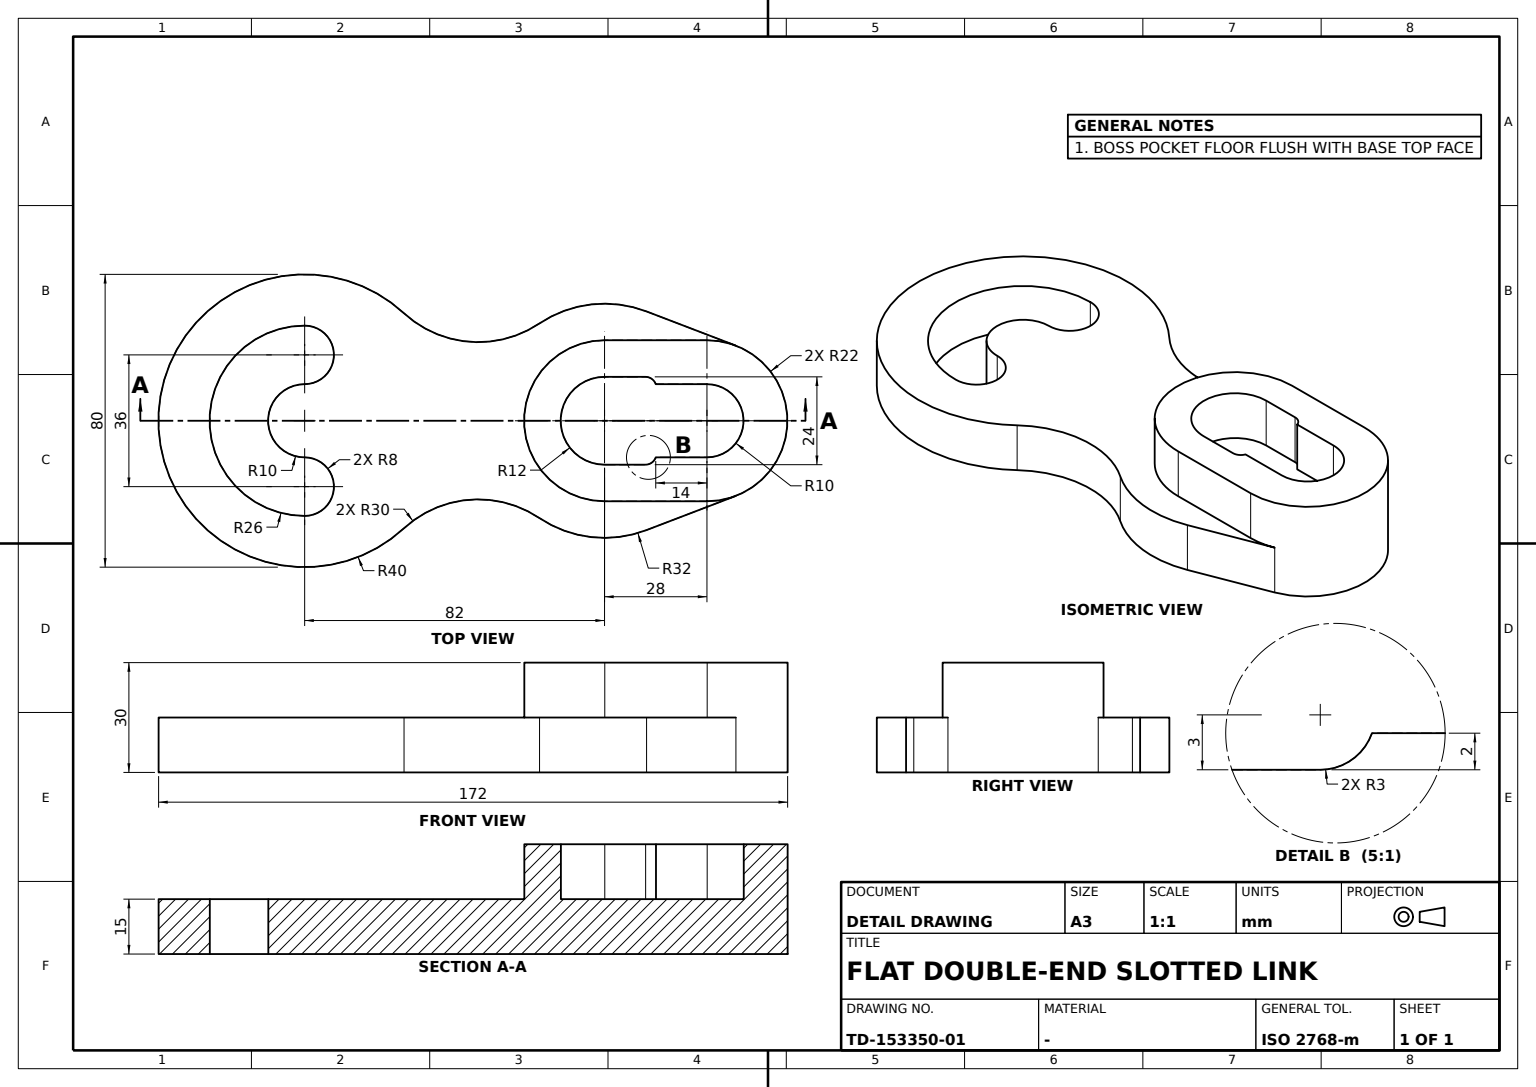
ISO-10303-21;
HEADER;
FILE_DESCRIPTION((''),'2;1');
FILE_NAME('','',(''),(''),'','','');
FILE_SCHEMA(('AUTOMOTIVE_DESIGN'));
ENDSEC;
DATA;
#1=APPLICATION_CONTEXT('');
#2=PRODUCT_CONTEXT('',#1,'mechanical');
#3=PRODUCT('','','',(#2));
#4=PRODUCT_DEFINITION_FORMATION('','',#3);
#5=PRODUCT_DEFINITION_CONTEXT('',#1,'design');
#6=PRODUCT_DEFINITION('','',#4,#5);
#7=PRODUCT_DEFINITION_SHAPE('','',#6);
#8=(LENGTH_UNIT()NAMED_UNIT(*)SI_UNIT(.MILLI.,.METRE.));
#9=(NAMED_UNIT(*)PLANE_ANGLE_UNIT()SI_UNIT($,.RADIAN.));
#10=(NAMED_UNIT(*)SI_UNIT($,.STERADIAN.)SOLID_ANGLE_UNIT());
#11=UNCERTAINTY_MEASURE_WITH_UNIT(LENGTH_MEASURE(0.005),#8,'distance_accuracy_value','');
#12=(GEOMETRIC_REPRESENTATION_CONTEXT(3)GLOBAL_UNCERTAINTY_ASSIGNED_CONTEXT((#11))GLOBAL_UNIT_ASSIGNED_CONTEXT((#8,#9,#10))REPRESENTATION_CONTEXT('',''));
#13=CARTESIAN_POINT('',(-10.,110.,15.));
#14=VERTEX_POINT('',#13);
#15=CARTESIAN_POINT('',(-10.,96.,15.));
#16=VERTEX_POINT('',#15);
#17=CARTESIAN_POINT('',(-10.,0.,15.));
#18=DIRECTION('',(0.,-1.,0.));
#19=VECTOR('',#18,1000.);
#20=LINE('',#17,#19);
#21=EDGE_CURVE('',#14,#16,#20,.T.);
#22=ORIENTED_EDGE('',*,*,#21,.T.);
#23=CARTESIAN_POINT('',(-10.,96.,0.));
#24=VERTEX_POINT('',#23);
#25=DIRECTION('',(0.,0.,1.));
#26=VECTOR('',#25,1000.);
#27=LINE('',#23,#26);
#28=EDGE_CURVE('',#24,#16,#27,.T.);
#29=ORIENTED_EDGE('',*,*,#28,.F.);
#30=CARTESIAN_POINT('',(-10.,110.,0.));
#31=VERTEX_POINT('',#30);
#32=CARTESIAN_POINT('',(-10.,0.,0.));
#33=LINE('',#32,#19);
#34=EDGE_CURVE('',#31,#24,#33,.T.);
#35=ORIENTED_EDGE('',*,*,#34,.F.);
#36=CARTESIAN_POINT('',(-10.,110.,7.5));
#37=LINE('',#36,#26);
#38=EDGE_CURVE('',#31,#14,#37,.T.);
#39=ORIENTED_EDGE('',*,*,#38,.T.);
#40=EDGE_LOOP('',(#22,#29,#35,#39));
#41=FACE_BOUND('',#40,.T.);
#42=DIRECTION('',(-1.,0.,0.));
#43=AXIS2_PLACEMENT_3D('',#30,#42,#18);
#44=PLANE('',#43);
#45=ADVANCED_FACE('',(#41),#44,.F.);
#46=CARTESIAN_POINT('',(12.,93.171573,0.));
#47=VERTEX_POINT('',#46);
#48=CARTESIAN_POINT('',(10.,96.,0.));
#49=VERTEX_POINT('',#48);
#50=CARTESIAN_POINT('',(9.,93.171573,0.));
#51=DIRECTION('',(1.,0.,0.));
#52=AXIS2_PLACEMENT_3D('',#50,#25,#51);
#53=CIRCLE('',#52,3.);
#54=EDGE_CURVE('',#47,#49,#53,.T.);
#55=ORIENTED_EDGE('',*,*,#54,.F.);
#56=CARTESIAN_POINT('',(12.,93.171573,15.));
#57=VERTEX_POINT('',#56);
#58=CARTESIAN_POINT('',(12.,93.171573,7.5));
#59=LINE('',#58,#26);
#60=EDGE_CURVE('',#47,#57,#59,.T.);
#61=ORIENTED_EDGE('',*,*,#60,.T.);
#62=CARTESIAN_POINT('',(10.,96.,15.));
#63=VERTEX_POINT('',#62);
#64=CARTESIAN_POINT('',(9.,93.171573,15.));
#65=AXIS2_PLACEMENT_3D('',#64,#25,#51);
#66=CIRCLE('',#65,3.);
#67=EDGE_CURVE('',#57,#63,#66,.T.);
#68=ORIENTED_EDGE('',*,*,#67,.T.);
#69=LINE('',#48,#26);
#70=EDGE_CURVE('',#49,#63,#69,.T.);
#71=ORIENTED_EDGE('',*,*,#70,.F.);
#72=EDGE_LOOP('',(#55,#61,#68,#71));
#73=FACE_BOUND('',#72,.T.);
#74=CARTESIAN_POINT('',(9.,93.171573,7.5));
#75=AXIS2_PLACEMENT_3D('',#74,#25,#51);
#76=CYLINDRICAL_SURFACE('',#75,3.);
#77=ADVANCED_FACE('',(#73),#76,.F.);
#78=ORIENTED_EDGE('',*,*,#34,.T.);
#79=CARTESIAN_POINT('',(-12.,93.171573,0.));
#80=VERTEX_POINT('',#79);
#81=CARTESIAN_POINT('',(-9.,93.171573,0.));
#82=AXIS2_PLACEMENT_3D('',#81,#25,#51);
#83=CIRCLE('',#82,3.);
#84=EDGE_CURVE('',#24,#80,#83,.T.);
#85=ORIENTED_EDGE('',*,*,#84,.T.);
#86=CARTESIAN_POINT('',(-12.,82.,0.));
#87=VERTEX_POINT('',#86);
#88=CARTESIAN_POINT('',(-12.,0.,0.));
#89=DIRECTION('',(0.,1.,0.));
#90=VECTOR('',#89,1000.);
#91=LINE('',#88,#90);
#92=EDGE_CURVE('',#87,#80,#91,.T.);
#93=ORIENTED_EDGE('',*,*,#92,.F.);
#94=CARTESIAN_POINT('',(12.,82.,0.));
#95=VERTEX_POINT('',#94);
#96=CARTESIAN_POINT('',(0.,82.,0.));
#97=AXIS2_PLACEMENT_3D('',#96,#25,#51);
#98=CIRCLE('',#97,12.);
#99=EDGE_CURVE('',#87,#95,#98,.T.);
#100=ORIENTED_EDGE('',*,*,#99,.T.);
#101=CARTESIAN_POINT('',(12.,0.,0.));
#102=LINE('',#101,#90);
#103=EDGE_CURVE('',#95,#47,#102,.T.);
#104=ORIENTED_EDGE('',*,*,#103,.T.);
#105=ORIENTED_EDGE('',*,*,#54,.T.);
#106=CARTESIAN_POINT('',(10.,110.,0.));
#107=VERTEX_POINT('',#106);
#108=CARTESIAN_POINT('',(10.,0.,0.));
#109=LINE('',#108,#19);
#110=EDGE_CURVE('',#107,#49,#109,.T.);
#111=ORIENTED_EDGE('',*,*,#110,.F.);
#112=CARTESIAN_POINT('',(0.,110.,0.));
#113=AXIS2_PLACEMENT_3D('',#112,#25,#51);
#114=CIRCLE('',#113,10.);
#115=EDGE_CURVE('',#107,#31,#114,.T.);
#116=ORIENTED_EDGE('',*,*,#115,.T.);
#117=EDGE_LOOP('',(#78,#85,#93,#100,#104,#105,#111,#116));
#118=FACE_BOUND('',#117,.T.);
#119=CARTESIAN_POINT('',(0.,0.,0.));
#120=AXIS2_PLACEMENT_3D('',#119,#25,#51);
#121=PLANE('',#120);
#122=ADVANCED_FACE('',(#118),#121,.T.);
#123=CARTESIAN_POINT('',(-29.413527,27.108014,0.));
#124=VERTEX_POINT('',#123);
#125=CARTESIAN_POINT('',(-26.567057,64.162077,0.));
#126=VERTEX_POINT('',#125);
#127=CARTESIAN_POINT('',(-51.473673,47.439024,0.));
#128=AXIS2_PLACEMENT_3D('',#127,#25,#51);
#129=CIRCLE('',#128,30.);
#130=EDGE_CURVE('',#124,#126,#129,.T.);
#131=ORIENTED_EDGE('',*,*,#130,.T.);
#132=CARTESIAN_POINT('',(-26.567057,64.162077,-15.));
#133=VERTEX_POINT('',#132);
#134=CARTESIAN_POINT('',(-26.567057,64.162077,-7.5));
#135=LINE('',#134,#26);
#136=EDGE_CURVE('',#126,#133,#135,.F.);
#137=ORIENTED_EDGE('',*,*,#136,.T.);
#138=CARTESIAN_POINT('',(-29.413527,27.108014,-15.));
#139=VERTEX_POINT('',#138);
#140=CARTESIAN_POINT('',(-51.473673,47.439024,-15.));
#141=AXIS2_PLACEMENT_3D('',#140,#25,#51);
#142=CIRCLE('',#141,30.);
#143=EDGE_CURVE('',#139,#133,#142,.T.);
#144=ORIENTED_EDGE('',*,*,#143,.F.);
#145=CARTESIAN_POINT('',(-29.413527,27.108014,-7.5));
#146=LINE('',#145,#26);
#147=EDGE_CURVE('',#124,#139,#146,.F.);
#148=ORIENTED_EDGE('',*,*,#147,.F.);
#149=EDGE_LOOP('',(#131,#137,#144,#148));
#150=FACE_BOUND('',#149,.T.);
#151=CARTESIAN_POINT('',(-51.473673,47.439024,-7.5));
#152=AXIS2_PLACEMENT_3D('',#151,#25,#51);
#153=CYLINDRICAL_SURFACE('',#152,30.);
#154=ADVANCED_FACE('',(#150),#153,.F.);
#155=CARTESIAN_POINT('',(29.889593,93.428571,0.));
#156=VERTEX_POINT('',#155);
#157=CARTESIAN_POINT('',(20.549095,117.857143,0.));
#158=VERTEX_POINT('',#157);
#159=DIRECTION('',(-0.357142857,0.934049774,0.));
#160=VECTOR('',#159,1000.);
#161=LINE('',#155,#160);
#162=EDGE_CURVE('',#156,#158,#161,.T.);
#163=ORIENTED_EDGE('',*,*,#162,.F.);
#164=CARTESIAN_POINT('',(29.889593,93.428571,-15.));
#165=VERTEX_POINT('',#164);
#166=CARTESIAN_POINT('',(29.889593,93.428571,-7.5));
#167=LINE('',#166,#26);
#168=EDGE_CURVE('',#156,#165,#167,.F.);
#169=ORIENTED_EDGE('',*,*,#168,.T.);
#170=CARTESIAN_POINT('',(20.549095,117.857143,-15.));
#171=VERTEX_POINT('',#170);
#172=LINE('',#164,#160);
#173=EDGE_CURVE('',#165,#171,#172,.T.);
#174=ORIENTED_EDGE('',*,*,#173,.T.);
#175=CARTESIAN_POINT('',(20.549095,117.857143,-7.5));
#176=LINE('',#175,#26);
#177=EDGE_CURVE('',#158,#171,#176,.F.);
#178=ORIENTED_EDGE('',*,*,#177,.F.);
#179=EDGE_LOOP('',(#163,#169,#174,#178));
#180=FACE_BOUND('',#179,.T.);
#181=DIRECTION('',(-0.934049774,-0.357142857,0.));
#182=AXIS2_PLACEMENT_3D('',#155,#181,#159);
#183=PLANE('',#182);
#184=ADVANCED_FACE('',(#180),#183,.F.);
#185=CARTESIAN_POINT('',(-22.,82.,0.));
#186=VERTEX_POINT('',#185);
#187=CARTESIAN_POINT('',(-22.,82.,15.));
#188=VERTEX_POINT('',#187);
#189=CARTESIAN_POINT('',(-22.,82.,7.5));
#190=LINE('',#189,#26);
#191=EDGE_CURVE('',#186,#188,#190,.T.);
#192=ORIENTED_EDGE('',*,*,#191,.T.);
#193=CARTESIAN_POINT('',(-22.,110.,15.));
#194=VERTEX_POINT('',#193);
#195=CARTESIAN_POINT('',(-22.,0.,15.));
#196=LINE('',#195,#90);
#197=EDGE_CURVE('',#188,#194,#196,.T.);
#198=ORIENTED_EDGE('',*,*,#197,.T.);
#199=CARTESIAN_POINT('',(-22.,110.,0.));
#200=VERTEX_POINT('',#199);
#201=CARTESIAN_POINT('',(-22.,110.,-7.5));
#202=LINE('',#201,#26);
#203=EDGE_CURVE('',#200,#194,#202,.T.);
#204=ORIENTED_EDGE('',*,*,#203,.F.);
#205=CARTESIAN_POINT('',(-22.,0.,0.));
#206=LINE('',#205,#90);
#207=EDGE_CURVE('',#186,#200,#206,.T.);
#208=ORIENTED_EDGE('',*,*,#207,.F.);
#209=EDGE_LOOP('',(#192,#198,#204,#208));
#210=FACE_BOUND('',#209,.T.);
#211=AXIS2_PLACEMENT_3D('',#185,#51,#89);
#212=PLANE('',#211);
#213=ADVANCED_FACE('',(#210),#212,.F.);
#214=ORIENTED_EDGE('',*,*,#168,.F.);
#215=CARTESIAN_POINT('',(26.567057,64.162077,0.));
#216=VERTEX_POINT('',#215);
#217=CIRCLE('',#97,32.);
#218=EDGE_CURVE('',#216,#156,#217,.T.);
#219=ORIENTED_EDGE('',*,*,#218,.F.);
#220=CARTESIAN_POINT('',(26.567057,64.162077,-15.));
#221=VERTEX_POINT('',#220);
#222=CARTESIAN_POINT('',(26.567057,64.162077,-7.5));
#223=LINE('',#222,#26);
#224=EDGE_CURVE('',#216,#221,#223,.F.);
#225=ORIENTED_EDGE('',*,*,#224,.T.);
#226=CARTESIAN_POINT('',(0.,82.,-15.));
#227=AXIS2_PLACEMENT_3D('',#226,#25,#51);
#228=CIRCLE('',#227,32.);
#229=EDGE_CURVE('',#221,#165,#228,.T.);
#230=ORIENTED_EDGE('',*,*,#229,.T.);
#231=EDGE_LOOP('',(#214,#219,#225,#230));
#232=FACE_BOUND('',#231,.T.);
#233=CARTESIAN_POINT('',(0.,82.,-7.5));
#234=AXIS2_PLACEMENT_3D('',#233,#25,#51);
#235=CYLINDRICAL_SURFACE('',#234,32.);
#236=ADVANCED_FACE('',(#232),#235,.T.);
#237=CARTESIAN_POINT('',(26.,0.,0.));
#238=VERTEX_POINT('',#237);
#239=CARTESIAN_POINT('',(26.,0.,-15.));
#240=VERTEX_POINT('',#239);
#241=CARTESIAN_POINT('',(26.,0.,-7.5));
#242=LINE('',#241,#26);
#243=EDGE_CURVE('',#238,#240,#242,.F.);
#244=ORIENTED_EDGE('',*,*,#243,.F.);
#245=VERTEX_POINT('',#108);
#246=CARTESIAN_POINT('',(18.,0.,0.));
#247=AXIS2_PLACEMENT_3D('',#246,#25,#51);
#248=CIRCLE('',#247,8.);
#249=EDGE_CURVE('',#238,#245,#248,.T.);
#250=ORIENTED_EDGE('',*,*,#249,.T.);
#251=CARTESIAN_POINT('',(10.,0.,-15.));
#252=VERTEX_POINT('',#251);
#253=CARTESIAN_POINT('',(10.,0.,-7.5));
#254=LINE('',#253,#26);
#255=EDGE_CURVE('',#245,#252,#254,.F.);
#256=ORIENTED_EDGE('',*,*,#255,.T.);
#257=CARTESIAN_POINT('',(18.,0.,-15.));
#258=AXIS2_PLACEMENT_3D('',#257,#25,#51);
#259=CIRCLE('',#258,8.);
#260=EDGE_CURVE('',#240,#252,#259,.T.);
#261=ORIENTED_EDGE('',*,*,#260,.F.);
#262=EDGE_LOOP('',(#244,#250,#256,#261));
#263=FACE_BOUND('',#262,.T.);
#264=CARTESIAN_POINT('',(18.,0.,-7.5));
#265=AXIS2_PLACEMENT_3D('',#264,#25,#51);
#266=CYLINDRICAL_SURFACE('',#265,8.);
#267=ADVANCED_FACE('',(#263),#266,.F.);
#268=ORIENTED_EDGE('',*,*,#191,.F.);
#269=CARTESIAN_POINT('',(22.,82.,0.));
#270=VERTEX_POINT('',#269);
#271=CIRCLE('',#97,22.);
#272=EDGE_CURVE('',#186,#270,#271,.T.);
#273=ORIENTED_EDGE('',*,*,#272,.T.);
#274=CARTESIAN_POINT('',(22.,82.,15.));
#275=VERTEX_POINT('',#274);
#276=CARTESIAN_POINT('',(22.,82.,7.5));
#277=LINE('',#276,#26);
#278=EDGE_CURVE('',#270,#275,#277,.T.);
#279=ORIENTED_EDGE('',*,*,#278,.T.);
#280=CARTESIAN_POINT('',(0.,82.,15.));
#281=AXIS2_PLACEMENT_3D('',#280,#25,#51);
#282=CIRCLE('',#281,22.);
#283=EDGE_CURVE('',#188,#275,#282,.T.);
#284=ORIENTED_EDGE('',*,*,#283,.F.);
#285=EDGE_LOOP('',(#268,#273,#279,#284));
#286=FACE_BOUND('',#285,.T.);
#287=CARTESIAN_POINT('',(0.,82.,7.5));
#288=AXIS2_PLACEMENT_3D('',#287,#25,#51);
#289=CYLINDRICAL_SURFACE('',#288,22.);
#290=ADVANCED_FACE('',(#286),#289,.T.);
#291=CARTESIAN_POINT('',(29.413527,27.108014,0.));
#292=VERTEX_POINT('',#291);
#293=CARTESIAN_POINT('',(29.413527,27.108014,-15.));
#294=VERTEX_POINT('',#293);
#295=CARTESIAN_POINT('',(29.413527,27.108014,-7.5));
#296=LINE('',#295,#26);
#297=EDGE_CURVE('',#292,#294,#296,.F.);
#298=ORIENTED_EDGE('',*,*,#297,.T.);
#299=CARTESIAN_POINT('',(51.473673,47.439024,-15.));
#300=AXIS2_PLACEMENT_3D('',#299,#25,#51);
#301=CIRCLE('',#300,30.);
#302=EDGE_CURVE('',#221,#294,#301,.T.);
#303=ORIENTED_EDGE('',*,*,#302,.F.);
#304=ORIENTED_EDGE('',*,*,#224,.F.);
#305=CARTESIAN_POINT('',(51.473673,47.439024,0.));
#306=AXIS2_PLACEMENT_3D('',#305,#25,#51);
#307=CIRCLE('',#306,30.);
#308=EDGE_CURVE('',#216,#292,#307,.T.);
#309=ORIENTED_EDGE('',*,*,#308,.T.);
#310=EDGE_LOOP('',(#298,#303,#304,#309));
#311=FACE_BOUND('',#310,.T.);
#312=CARTESIAN_POINT('',(51.473673,47.439024,-7.5));
#313=AXIS2_PLACEMENT_3D('',#312,#25,#51);
#314=CYLINDRICAL_SURFACE('',#313,30.);
#315=ADVANCED_FACE('',(#311),#314,.F.);
#316=ORIENTED_EDGE('',*,*,#110,.T.);
#317=ORIENTED_EDGE('',*,*,#70,.T.);
#318=CARTESIAN_POINT('',(10.,110.,15.));
#319=VERTEX_POINT('',#318);
#320=CARTESIAN_POINT('',(10.,0.,15.));
#321=LINE('',#320,#19);
#322=EDGE_CURVE('',#319,#63,#321,.T.);
#323=ORIENTED_EDGE('',*,*,#322,.F.);
#324=CARTESIAN_POINT('',(10.,110.,7.5));
#325=LINE('',#324,#26);
#326=EDGE_CURVE('',#107,#319,#325,.T.);
#327=ORIENTED_EDGE('',*,*,#326,.F.);
#328=EDGE_LOOP('',(#316,#317,#323,#327));
#329=FACE_BOUND('',#328,.T.);
#330=AXIS2_PLACEMENT_3D('',#106,#42,#18);
#331=PLANE('',#330);
#332=ADVANCED_FACE('',(#329),#331,.T.);
#333=ORIENTED_EDGE('',*,*,#103,.F.);
#334=CARTESIAN_POINT('',(12.,82.,15.));
#335=VERTEX_POINT('',#334);
#336=CARTESIAN_POINT('',(12.,82.,7.5));
#337=LINE('',#336,#26);
#338=EDGE_CURVE('',#95,#335,#337,.T.);
#339=ORIENTED_EDGE('',*,*,#338,.T.);
#340=CARTESIAN_POINT('',(12.,0.,15.));
#341=LINE('',#340,#90);
#342=EDGE_CURVE('',#335,#57,#341,.T.);
#343=ORIENTED_EDGE('',*,*,#342,.T.);
#344=ORIENTED_EDGE('',*,*,#60,.F.);
#345=EDGE_LOOP('',(#333,#339,#343,#344));
#346=FACE_BOUND('',#345,.T.);
#347=AXIS2_PLACEMENT_3D('',#94,#51,#89);
#348=PLANE('',#347);
#349=ADVANCED_FACE('',(#346),#348,.F.);
#350=VERTEX_POINT('',#32);
#351=CARTESIAN_POINT('',(-10.,0.,-15.));
#352=VERTEX_POINT('',#351);
#353=CARTESIAN_POINT('',(-10.,0.,-7.5));
#354=LINE('',#353,#26);
#355=EDGE_CURVE('',#350,#352,#354,.F.);
#356=ORIENTED_EDGE('',*,*,#355,.T.);
#357=CARTESIAN_POINT('',(0.,0.,-15.));
#358=AXIS2_PLACEMENT_3D('',#357,#25,#51);
#359=CIRCLE('',#358,10.);
#360=EDGE_CURVE('',#352,#252,#359,.T.);
#361=ORIENTED_EDGE('',*,*,#360,.T.);
#362=ORIENTED_EDGE('',*,*,#255,.F.);
#363=CIRCLE('',#120,10.);
#364=EDGE_CURVE('',#350,#245,#363,.T.);
#365=ORIENTED_EDGE('',*,*,#364,.F.);
#366=EDGE_LOOP('',(#356,#361,#362,#365));
#367=FACE_BOUND('',#366,.T.);
#368=CARTESIAN_POINT('',(0.,0.,-7.5));
#369=AXIS2_PLACEMENT_3D('',#368,#25,#51);
#370=CYLINDRICAL_SURFACE('',#369,10.);
#371=ADVANCED_FACE('',(#367),#370,.T.);
#372=ORIENTED_EDGE('',*,*,#21,.F.);
#373=CARTESIAN_POINT('',(0.,110.,15.));
#374=AXIS2_PLACEMENT_3D('',#373,#25,#51);
#375=CIRCLE('',#374,10.);
#376=EDGE_CURVE('',#319,#14,#375,.T.);
#377=ORIENTED_EDGE('',*,*,#376,.F.);
#378=ORIENTED_EDGE('',*,*,#322,.T.);
#379=ORIENTED_EDGE('',*,*,#67,.F.);
#380=ORIENTED_EDGE('',*,*,#342,.F.);
#381=CARTESIAN_POINT('',(-12.,82.,15.));
#382=VERTEX_POINT('',#381);
#383=CIRCLE('',#281,12.);
#384=EDGE_CURVE('',#382,#335,#383,.T.);
#385=ORIENTED_EDGE('',*,*,#384,.F.);
#386=CARTESIAN_POINT('',(-12.,93.171573,15.));
#387=VERTEX_POINT('',#386);
#388=CARTESIAN_POINT('',(-12.,0.,15.));
#389=LINE('',#388,#90);
#390=EDGE_CURVE('',#382,#387,#389,.T.);
#391=ORIENTED_EDGE('',*,*,#390,.T.);
#392=CARTESIAN_POINT('',(-9.,93.171573,15.));
#393=AXIS2_PLACEMENT_3D('',#392,#25,#51);
#394=CIRCLE('',#393,3.);
#395=EDGE_CURVE('',#16,#387,#394,.T.);
#396=ORIENTED_EDGE('',*,*,#395,.F.);
#397=EDGE_LOOP('',(#372,#377,#378,#379,#380,#385,#391,#396));
#398=FACE_BOUND('',#397,.T.);
#399=ORIENTED_EDGE('',*,*,#197,.F.);
#400=ORIENTED_EDGE('',*,*,#283,.T.);
#401=CARTESIAN_POINT('',(22.,110.,15.));
#402=VERTEX_POINT('',#401);
#403=CARTESIAN_POINT('',(22.,0.,15.));
#404=LINE('',#403,#19);
#405=EDGE_CURVE('',#402,#275,#404,.T.);
#406=ORIENTED_EDGE('',*,*,#405,.F.);
#407=CIRCLE('',#374,22.);
#408=EDGE_CURVE('',#402,#194,#407,.T.);
#409=ORIENTED_EDGE('',*,*,#408,.T.);
#410=EDGE_LOOP('',(#399,#400,#406,#409));
#411=FACE_BOUND('',#410,.T.);
#412=CARTESIAN_POINT('',(0.,0.,15.));
#413=AXIS2_PLACEMENT_3D('',#412,#25,#51);
#414=PLANE('',#413);
#415=ADVANCED_FACE('',(#398,#411),#414,.T.);
#416=CARTESIAN_POINT('',(-12.,82.,7.5));
#417=LINE('',#416,#26);
#418=EDGE_CURVE('',#87,#382,#417,.T.);
#419=ORIENTED_EDGE('',*,*,#418,.T.);
#420=ORIENTED_EDGE('',*,*,#384,.T.);
#421=ORIENTED_EDGE('',*,*,#338,.F.);
#422=ORIENTED_EDGE('',*,*,#99,.F.);
#423=EDGE_LOOP('',(#419,#420,#421,#422));
#424=FACE_BOUND('',#423,.T.);
#425=CYLINDRICAL_SURFACE('',#288,12.);
#426=ADVANCED_FACE('',(#424),#425,.F.);
#427=ORIENTED_EDGE('',*,*,#326,.T.);
#428=ORIENTED_EDGE('',*,*,#376,.T.);
#429=ORIENTED_EDGE('',*,*,#38,.F.);
#430=ORIENTED_EDGE('',*,*,#115,.F.);
#431=EDGE_LOOP('',(#427,#428,#429,#430));
#432=FACE_BOUND('',#431,.T.);
#433=CARTESIAN_POINT('',(0.,110.,7.5));
#434=AXIS2_PLACEMENT_3D('',#433,#25,#51);
#435=CYLINDRICAL_SURFACE('',#434,10.);
#436=ADVANCED_FACE('',(#432),#435,.F.);
#437=ORIENTED_EDGE('',*,*,#92,.T.);
#438=CARTESIAN_POINT('',(-12.,93.171573,7.5));
#439=LINE('',#438,#26);
#440=EDGE_CURVE('',#80,#387,#439,.T.);
#441=ORIENTED_EDGE('',*,*,#440,.T.);
#442=ORIENTED_EDGE('',*,*,#390,.F.);
#443=ORIENTED_EDGE('',*,*,#418,.F.);
#444=EDGE_LOOP('',(#437,#441,#442,#443));
#445=FACE_BOUND('',#444,.T.);
#446=AXIS2_PLACEMENT_3D('',#86,#51,#89);
#447=PLANE('',#446);
#448=ADVANCED_FACE('',(#445),#447,.T.);
#449=CIRCLE('',#120,40.);
#450=EDGE_CURVE('',#124,#292,#449,.T.);
#451=ORIENTED_EDGE('',*,*,#450,.F.);
#452=ORIENTED_EDGE('',*,*,#147,.T.);
#453=CIRCLE('',#358,40.);
#454=EDGE_CURVE('',#139,#294,#453,.T.);
#455=ORIENTED_EDGE('',*,*,#454,.T.);
#456=ORIENTED_EDGE('',*,*,#297,.F.);
#457=EDGE_LOOP('',(#451,#452,#455,#456));
#458=FACE_BOUND('',#457,.T.);
#459=CYLINDRICAL_SURFACE('',#369,40.);
#460=ADVANCED_FACE('',(#458),#459,.T.);
#461=CARTESIAN_POINT('',(-26.,0.,-15.));
#462=VERTEX_POINT('',#461);
#463=CIRCLE('',#358,26.);
#464=EDGE_CURVE('',#462,#240,#463,.T.);
#465=ORIENTED_EDGE('',*,*,#464,.F.);
#466=CARTESIAN_POINT('',(-26.,0.,0.));
#467=VERTEX_POINT('',#466);
#468=CARTESIAN_POINT('',(-26.,0.,-7.5));
#469=LINE('',#468,#26);
#470=EDGE_CURVE('',#467,#462,#469,.F.);
#471=ORIENTED_EDGE('',*,*,#470,.F.);
#472=CIRCLE('',#120,26.);
#473=EDGE_CURVE('',#467,#238,#472,.T.);
#474=ORIENTED_EDGE('',*,*,#473,.T.);
#475=ORIENTED_EDGE('',*,*,#243,.T.);
#476=EDGE_LOOP('',(#465,#471,#474,#475));
#477=FACE_BOUND('',#476,.T.);
#478=CYLINDRICAL_SURFACE('',#369,26.);
#479=ADVANCED_FACE('',(#477),#478,.F.);
#480=ORIENTED_EDGE('',*,*,#84,.F.);
#481=ORIENTED_EDGE('',*,*,#28,.T.);
#482=ORIENTED_EDGE('',*,*,#395,.T.);
#483=ORIENTED_EDGE('',*,*,#440,.F.);
#484=EDGE_LOOP('',(#480,#481,#482,#483));
#485=FACE_BOUND('',#484,.T.);
#486=CARTESIAN_POINT('',(-9.,93.171573,7.5));
#487=AXIS2_PLACEMENT_3D('',#486,#25,#51);
#488=CYLINDRICAL_SURFACE('',#487,3.);
#489=ADVANCED_FACE('',(#485),#488,.F.);
#490=CARTESIAN_POINT('',(-29.889593,93.428571,0.));
#491=VERTEX_POINT('',#490);
#492=EDGE_CURVE('',#491,#126,#217,.T.);
#493=ORIENTED_EDGE('',*,*,#492,.T.);
#494=ORIENTED_EDGE('',*,*,#130,.F.);
#495=ORIENTED_EDGE('',*,*,#450,.T.);
#496=ORIENTED_EDGE('',*,*,#308,.F.);
#497=ORIENTED_EDGE('',*,*,#218,.T.);
#498=ORIENTED_EDGE('',*,*,#162,.T.);
#499=CARTESIAN_POINT('',(22.,110.,0.));
#500=VERTEX_POINT('',#499);
#501=CIRCLE('',#113,22.);
#502=EDGE_CURVE('',#500,#158,#501,.T.);
#503=ORIENTED_EDGE('',*,*,#502,.F.);
#504=CARTESIAN_POINT('',(22.,0.,0.));
#505=LINE('',#504,#19);
#506=EDGE_CURVE('',#500,#270,#505,.T.);
#507=ORIENTED_EDGE('',*,*,#506,.T.);
#508=ORIENTED_EDGE('',*,*,#272,.F.);
#509=ORIENTED_EDGE('',*,*,#207,.T.);
#510=CARTESIAN_POINT('',(-20.549095,117.857143,0.));
#511=VERTEX_POINT('',#510);
#512=EDGE_CURVE('',#511,#200,#501,.T.);
#513=ORIENTED_EDGE('',*,*,#512,.F.);
#514=DIRECTION('',(0.357142857,0.934049774,0.));
#515=VECTOR('',#514,1000.);
#516=LINE('',#490,#515);
#517=EDGE_CURVE('',#491,#511,#516,.T.);
#518=ORIENTED_EDGE('',*,*,#517,.F.);
#519=EDGE_LOOP('',(#493,#494,#495,#496,#497,#498,#503,#507,#508,#509,#513,#518));
#520=FACE_BOUND('',#519,.T.);
#521=ORIENTED_EDGE('',*,*,#473,.F.);
#522=CARTESIAN_POINT('',(-18.,0.,0.));
#523=AXIS2_PLACEMENT_3D('',#522,#25,#51);
#524=CIRCLE('',#523,8.);
#525=EDGE_CURVE('',#350,#467,#524,.T.);
#526=ORIENTED_EDGE('',*,*,#525,.F.);
#527=ORIENTED_EDGE('',*,*,#364,.T.);
#528=ORIENTED_EDGE('',*,*,#249,.F.);
#529=EDGE_LOOP('',(#521,#526,#527,#528));
#530=FACE_BOUND('',#529,.T.);
#531=ADVANCED_FACE('',(#520,#530),#121,.T.);
#532=CARTESIAN_POINT('',(-20.549095,117.857143,-15.));
#533=VERTEX_POINT('',#532);
#534=CARTESIAN_POINT('',(-20.549095,117.857143,-7.5));
#535=LINE('',#534,#26);
#536=EDGE_CURVE('',#511,#533,#535,.F.);
#537=ORIENTED_EDGE('',*,*,#536,.T.);
#538=CARTESIAN_POINT('',(-29.889593,93.428571,-15.));
#539=VERTEX_POINT('',#538);
#540=LINE('',#538,#515);
#541=EDGE_CURVE('',#539,#533,#540,.T.);
#542=ORIENTED_EDGE('',*,*,#541,.F.);
#543=CARTESIAN_POINT('',(-29.889593,93.428571,-7.5));
#544=LINE('',#543,#26);
#545=EDGE_CURVE('',#491,#539,#544,.F.);
#546=ORIENTED_EDGE('',*,*,#545,.F.);
#547=ORIENTED_EDGE('',*,*,#517,.T.);
#548=EDGE_LOOP('',(#537,#542,#546,#547));
#549=FACE_BOUND('',#548,.T.);
#550=DIRECTION('',(-0.934049774,0.357142857,0.));
#551=AXIS2_PLACEMENT_3D('',#490,#550,#514);
#552=PLANE('',#551);
#553=ADVANCED_FACE('',(#549),#552,.T.);
#554=ORIENTED_EDGE('',*,*,#136,.F.);
#555=ORIENTED_EDGE('',*,*,#492,.F.);
#556=ORIENTED_EDGE('',*,*,#545,.T.);
#557=EDGE_CURVE('',#539,#133,#228,.T.);
#558=ORIENTED_EDGE('',*,*,#557,.T.);
#559=EDGE_LOOP('',(#554,#555,#556,#558));
#560=FACE_BOUND('',#559,.T.);
#561=ADVANCED_FACE('',(#560),#235,.T.);
#562=ORIENTED_EDGE('',*,*,#405,.T.);
#563=ORIENTED_EDGE('',*,*,#278,.F.);
#564=ORIENTED_EDGE('',*,*,#506,.F.);
#565=CARTESIAN_POINT('',(22.,110.,-7.5));
#566=LINE('',#565,#26);
#567=EDGE_CURVE('',#500,#402,#566,.T.);
#568=ORIENTED_EDGE('',*,*,#567,.T.);
#569=EDGE_LOOP('',(#562,#563,#564,#568));
#570=FACE_BOUND('',#569,.T.);
#571=AXIS2_PLACEMENT_3D('',#499,#42,#18);
#572=PLANE('',#571);
#573=ADVANCED_FACE('',(#570),#572,.F.);
#574=ORIENTED_EDGE('',*,*,#541,.T.);
#575=CARTESIAN_POINT('',(0.,110.,-15.));
#576=AXIS2_PLACEMENT_3D('',#575,#25,#51);
#577=CIRCLE('',#576,22.);
#578=EDGE_CURVE('',#171,#533,#577,.T.);
#579=ORIENTED_EDGE('',*,*,#578,.F.);
#580=ORIENTED_EDGE('',*,*,#173,.F.);
#581=ORIENTED_EDGE('',*,*,#229,.F.);
#582=ORIENTED_EDGE('',*,*,#302,.T.);
#583=ORIENTED_EDGE('',*,*,#454,.F.);
#584=ORIENTED_EDGE('',*,*,#143,.T.);
#585=ORIENTED_EDGE('',*,*,#557,.F.);
#586=EDGE_LOOP('',(#574,#579,#580,#581,#582,#583,#584,#585));
#587=FACE_BOUND('',#586,.T.);
#588=ORIENTED_EDGE('',*,*,#464,.T.);
#589=ORIENTED_EDGE('',*,*,#260,.T.);
#590=ORIENTED_EDGE('',*,*,#360,.F.);
#591=CARTESIAN_POINT('',(-18.,0.,-15.));
#592=AXIS2_PLACEMENT_3D('',#591,#25,#51);
#593=CIRCLE('',#592,8.);
#594=EDGE_CURVE('',#352,#462,#593,.T.);
#595=ORIENTED_EDGE('',*,*,#594,.T.);
#596=EDGE_LOOP('',(#588,#589,#590,#595));
#597=FACE_BOUND('',#596,.T.);
#598=PLANE('',#358);
#599=ADVANCED_FACE('',(#587,#597),#598,.F.);
#600=ORIENTED_EDGE('',*,*,#578,.T.);
#601=ORIENTED_EDGE('',*,*,#536,.F.);
#602=ORIENTED_EDGE('',*,*,#512,.T.);
#603=ORIENTED_EDGE('',*,*,#203,.T.);
#604=ORIENTED_EDGE('',*,*,#408,.F.);
#605=ORIENTED_EDGE('',*,*,#567,.F.);
#606=ORIENTED_EDGE('',*,*,#502,.T.);
#607=ORIENTED_EDGE('',*,*,#177,.T.);
#608=EDGE_LOOP('',(#600,#601,#602,#603,#604,#605,#606,#607));
#609=FACE_BOUND('',#608,.T.);
#610=CARTESIAN_POINT('',(0.,110.,-7.5));
#611=AXIS2_PLACEMENT_3D('',#610,#25,#51);
#612=CYLINDRICAL_SURFACE('',#611,22.);
#613=ADVANCED_FACE('',(#609),#612,.T.);
#614=ORIENTED_EDGE('',*,*,#470,.T.);
#615=ORIENTED_EDGE('',*,*,#594,.F.);
#616=ORIENTED_EDGE('',*,*,#355,.F.);
#617=ORIENTED_EDGE('',*,*,#525,.T.);
#618=EDGE_LOOP('',(#614,#615,#616,#617));
#619=FACE_BOUND('',#618,.T.);
#620=CARTESIAN_POINT('',(-18.,0.,-7.5));
#621=AXIS2_PLACEMENT_3D('',#620,#25,#51);
#622=CYLINDRICAL_SURFACE('',#621,8.);
#623=ADVANCED_FACE('',(#619),#622,.F.);
#624=CLOSED_SHELL('',(#45,#77,#122,#154,#184,#213,#236,#267,#290,#315,#332,#349,#371,#415,#426,#436,#448,#460,#479,#489,#531,#553,#561,#573,#599,#613,#623));
#625=MANIFOLD_SOLID_BREP('',#624);
#626=ADVANCED_BREP_SHAPE_REPRESENTATION('',(#625),#12);
#627=SHAPE_DEFINITION_REPRESENTATION(#7,#626);
ENDSEC;
END-ISO-10303-21;
